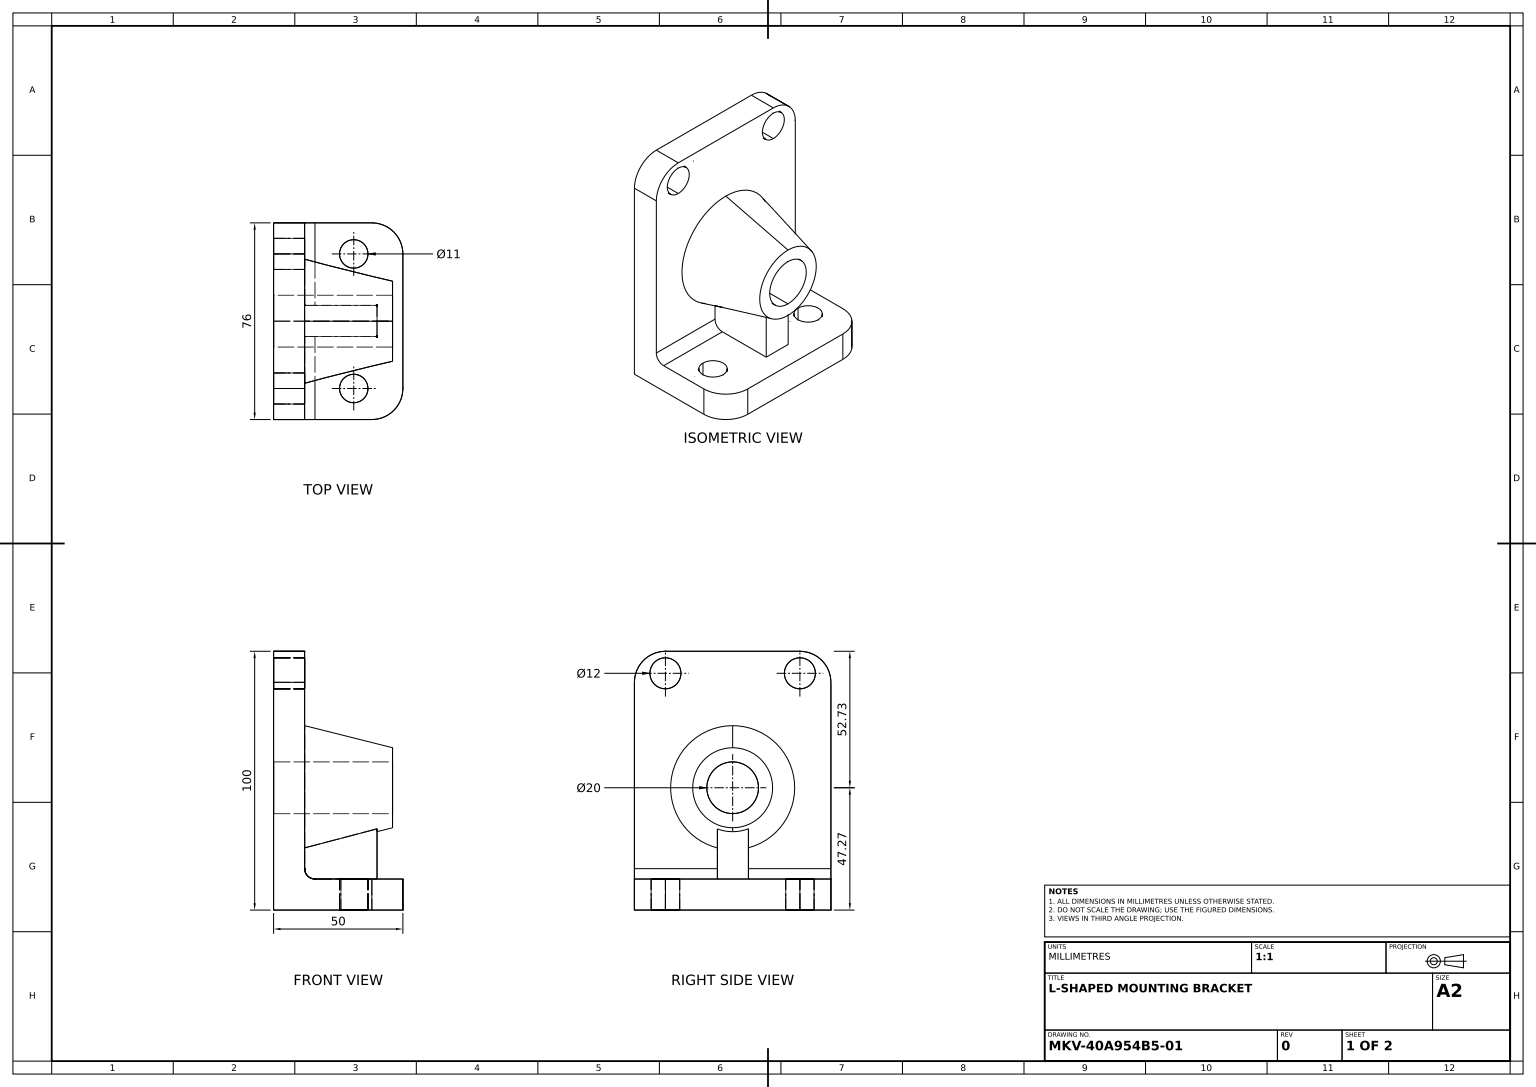
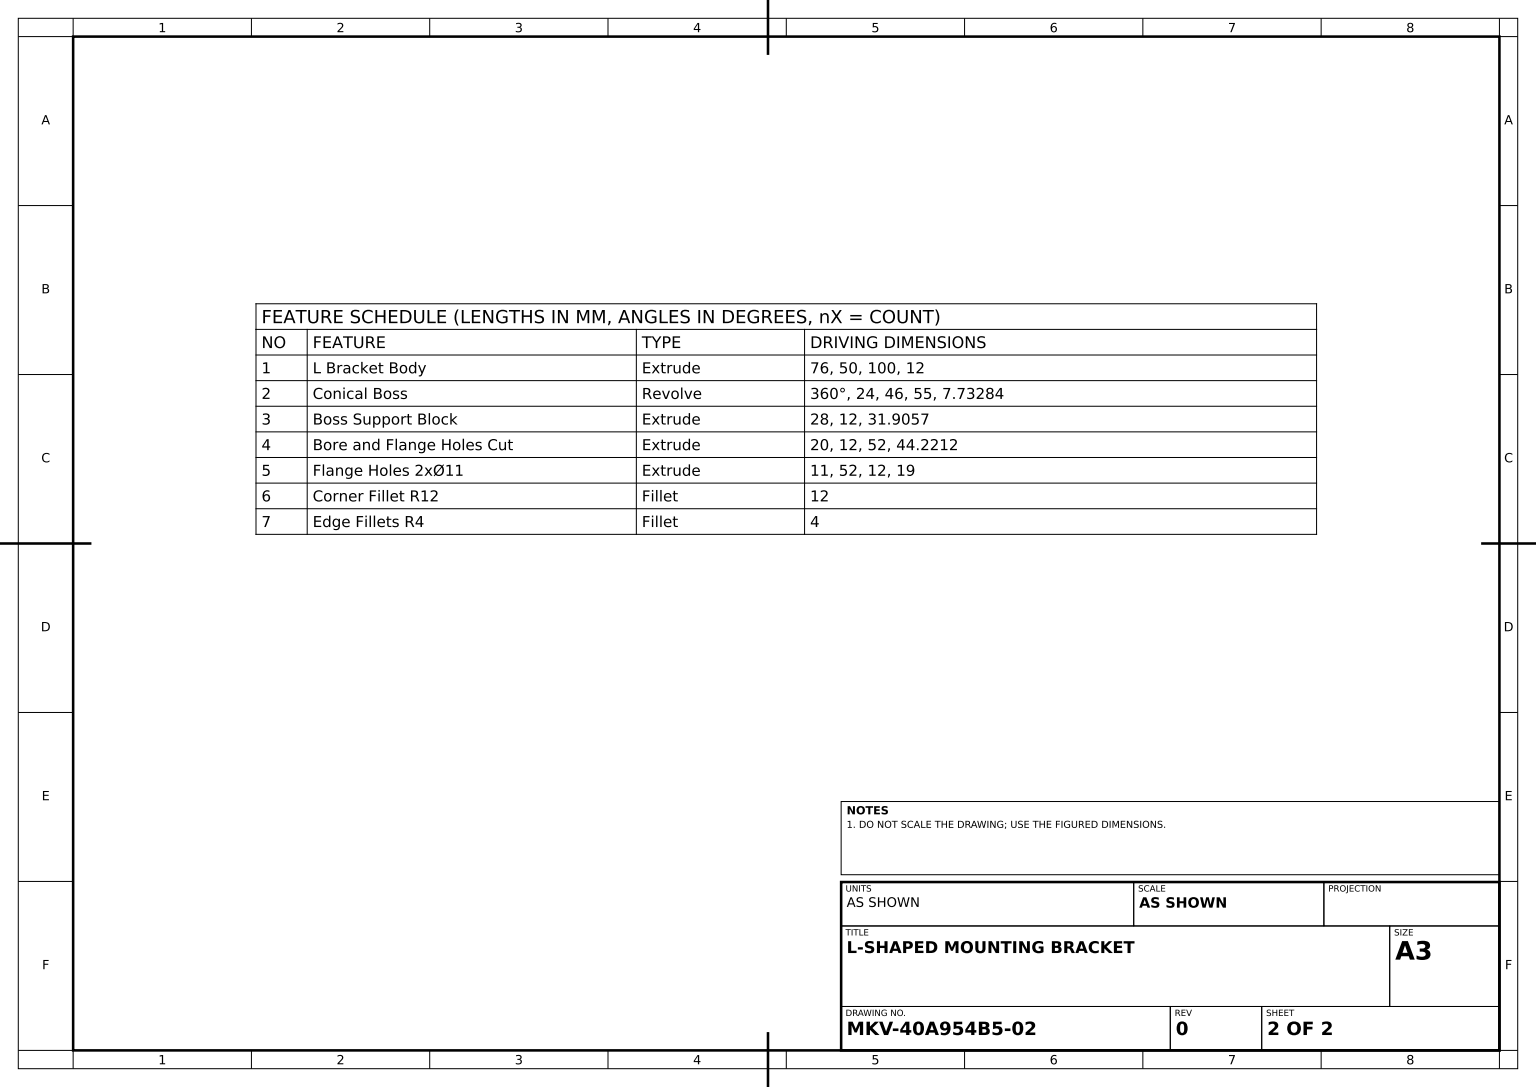
ISO-10303-21;
HEADER;
FILE_DESCRIPTION((''),'2;1');
FILE_NAME('','',(''),(''),'','','');
FILE_SCHEMA(('AUTOMOTIVE_DESIGN'));
ENDSEC;
DATA;
#1=APPLICATION_CONTEXT('');
#2=PRODUCT_CONTEXT('',#1,'mechanical');
#3=PRODUCT('','','',(#2));
#4=PRODUCT_DEFINITION_FORMATION('','',#3);
#5=PRODUCT_DEFINITION_CONTEXT('',#1,'design');
#6=PRODUCT_DEFINITION('','',#4,#5);
#7=PRODUCT_DEFINITION_SHAPE('','',#6);
#8=(LENGTH_UNIT()NAMED_UNIT(*)SI_UNIT(.MILLI.,.METRE.));
#9=(NAMED_UNIT(*)PLANE_ANGLE_UNIT()SI_UNIT($,.RADIAN.));
#10=(NAMED_UNIT(*)SI_UNIT($,.STERADIAN.)SOLID_ANGLE_UNIT());
#11=UNCERTAINTY_MEASURE_WITH_UNIT(LENGTH_MEASURE(1.E-05),#8,'distance_accuracy_value','');
#12=(GEOMETRIC_REPRESENTATION_CONTEXT(3)GLOBAL_UNCERTAINTY_ASSIGNED_CONTEXT((#11))GLOBAL_UNIT_ASSIGNED_CONTEXT((#8,#9,#10))REPRESENTATION_CONTEXT('',''));
#13=CARTESIAN_POINT('',(0.,57.267161,0.));
#14=VERTEX_POINT('',#13);
#15=CARTESIAN_POINT('',(46.,57.267161,0.));
#16=VERTEX_POINT('',#15);
#17=DIRECTION('',(1.,0.,0.));
#18=VECTOR('',#17,1000.);
#19=LINE('',#13,#18);
#20=EDGE_CURVE('',#14,#16,#19,.T.);
#21=ORIENTED_EDGE('',*,*,#20,.T.);
#22=CARTESIAN_POINT('',(46.,37.267161,0.));
#23=VERTEX_POINT('',#22);
#24=CARTESIAN_POINT('',(46.,47.267161,0.));
#25=DIRECTION('',(0.,1.,0.));
#26=AXIS2_PLACEMENT_3D('',#24,#17,#25);
#27=CIRCLE('',#26,10.);
#28=EDGE_CURVE('',#16,#23,#27,.T.);
#29=ORIENTED_EDGE('',*,*,#28,.T.);
#30=CARTESIAN_POINT('',(0.,37.267161,0.));
#31=VERTEX_POINT('',#30);
#32=LINE('',#30,#18);
#33=EDGE_CURVE('',#31,#23,#32,.T.);
#34=ORIENTED_EDGE('',*,*,#33,.F.);
#35=CARTESIAN_POINT('',(0.,47.267161,0.));
#36=AXIS2_PLACEMENT_3D('',#35,#17,#25);
#37=CIRCLE('',#36,10.);
#38=EDGE_CURVE('',#14,#31,#37,.T.);
#39=ORIENTED_EDGE('',*,*,#38,.F.);
#40=EDGE_LOOP('',(#21,#29,#34,#39));
#41=FACE_OUTER_BOUND('',#40,.T.);
#42=CYLINDRICAL_SURFACE('',#36,10.);
#43=ADVANCED_FACE('',(#41),#42,.F.);
#44=CARTESIAN_POINT('',(36.5,12.,-26.));
#45=VERTEX_POINT('',#44);
#46=CARTESIAN_POINT('',(25.5,12.,-26.));
#47=VERTEX_POINT('',#46);
#48=CARTESIAN_POINT('',(31.,12.,-26.));
#49=DIRECTION('',(-1.,0.,0.));
#50=AXIS2_PLACEMENT_3D('',#48,#25,#49);
#51=CIRCLE('',#50,5.5);
#52=EDGE_CURVE('',#45,#47,#51,.T.);
#53=ORIENTED_EDGE('',*,*,#52,.F.);
#54=EDGE_CURVE('',#47,#45,#51,.T.);
#55=ORIENTED_EDGE('',*,*,#54,.F.);
#56=EDGE_LOOP('',(#53,#55));
#57=FACE_BOUND('',#56,.T.);
#58=CARTESIAN_POINT('',(38.,12.,-38.));
#59=VERTEX_POINT('',#58);
#60=CARTESIAN_POINT('',(16.,12.,-38.));
#61=VERTEX_POINT('',#60);
#62=CARTESIAN_POINT('',(50.,12.,-38.));
#63=VECTOR('',#49,1000.);
#64=LINE('',#62,#63);
#65=EDGE_CURVE('',#59,#61,#64,.T.);
#66=ORIENTED_EDGE('',*,*,#65,.T.);
#67=CARTESIAN_POINT('',(16.,12.,-6.094262));
#68=VERTEX_POINT('',#67);
#69=DIRECTION('',(0.,0.,1.));
#70=VECTOR('',#69,1000.);
#71=LINE('',#67,#70);
#72=EDGE_CURVE('',#61,#68,#71,.T.);
#73=ORIENTED_EDGE('',*,*,#72,.T.);
#74=CARTESIAN_POINT('',(40.,12.,-6.094262));
#75=VERTEX_POINT('',#74);
#76=CARTESIAN_POINT('',(12.,12.,-6.094262));
#77=LINE('',#76,#18);
#78=EDGE_CURVE('',#68,#75,#77,.T.);
#79=ORIENTED_EDGE('',*,*,#78,.T.);
#80=CARTESIAN_POINT('',(40.,12.,5.905738));
#81=VERTEX_POINT('',#80);
#82=DIRECTION('',(0.,0.,-1.));
#83=VECTOR('',#82,1000.);
#84=LINE('',#80,#83);
#85=EDGE_CURVE('',#81,#75,#84,.T.);
#86=ORIENTED_EDGE('',*,*,#85,.F.);
#87=CARTESIAN_POINT('',(16.,12.,5.905738));
#88=VERTEX_POINT('',#87);
#89=CARTESIAN_POINT('',(12.,12.,5.905738));
#90=LINE('',#89,#18);
#91=EDGE_CURVE('',#88,#81,#90,.T.);
#92=ORIENTED_EDGE('',*,*,#91,.F.);
#93=CARTESIAN_POINT('',(16.,12.,38.));
#94=VERTEX_POINT('',#93);
#95=LINE('',#93,#70);
#96=EDGE_CURVE('',#88,#94,#95,.T.);
#97=ORIENTED_EDGE('',*,*,#96,.T.);
#98=CARTESIAN_POINT('',(38.,12.,38.));
#99=VERTEX_POINT('',#98);
#100=CARTESIAN_POINT('',(50.,12.,38.));
#101=LINE('',#100,#63);
#102=EDGE_CURVE('',#99,#94,#101,.T.);
#103=ORIENTED_EDGE('',*,*,#102,.F.);
#104=CARTESIAN_POINT('',(50.,12.,26.));
#105=VERTEX_POINT('',#104);
#106=CARTESIAN_POINT('',(38.,12.,26.));
#107=AXIS2_PLACEMENT_3D('',#106,#25,#17);
#108=CIRCLE('',#107,12.);
#109=EDGE_CURVE('',#99,#105,#108,.T.);
#110=ORIENTED_EDGE('',*,*,#109,.T.);
#111=CARTESIAN_POINT('',(50.,12.,-26.));
#112=VERTEX_POINT('',#111);
#113=LINE('',#100,#83);
#114=EDGE_CURVE('',#105,#112,#113,.T.);
#115=ORIENTED_EDGE('',*,*,#114,.T.);
#116=CARTESIAN_POINT('',(38.,12.,-26.));
#117=AXIS2_PLACEMENT_3D('',#116,#25,#17);
#118=CIRCLE('',#117,12.);
#119=EDGE_CURVE('',#112,#59,#118,.T.);
#120=ORIENTED_EDGE('',*,*,#119,.T.);
#121=EDGE_LOOP('',(#66,#73,#79,#86,#92,#97,#103,#110,#115,#120));
#122=FACE_OUTER_BOUND('',#121,.T.);
#123=CARTESIAN_POINT('',(36.5,12.,26.));
#124=VERTEX_POINT('',#123);
#125=CARTESIAN_POINT('',(25.5,12.,26.));
#126=VERTEX_POINT('',#125);
#127=CARTESIAN_POINT('',(31.,12.,26.));
#128=AXIS2_PLACEMENT_3D('',#127,#25,#49);
#129=CIRCLE('',#128,5.5);
#130=EDGE_CURVE('',#124,#126,#129,.T.);
#131=ORIENTED_EDGE('',*,*,#130,.F.);
#132=EDGE_CURVE('',#126,#124,#129,.T.);
#133=ORIENTED_EDGE('',*,*,#132,.F.);
#134=EDGE_LOOP('',(#131,#133));
#135=FACE_BOUND('',#134,.T.);
#136=DIRECTION('',(0.,-1.,0.));
#137=AXIS2_PLACEMENT_3D('',#100,#136,#17);
#138=PLANE('',#137);
#139=ADVANCED_FACE('',(#57,#122,#135),#138,.F.);
#140=CARTESIAN_POINT('',(50.,0.,-26.));
#141=VERTEX_POINT('',#140);
#142=VECTOR('',#25,1000.);
#143=LINE('',#140,#142);
#144=EDGE_CURVE('',#141,#112,#143,.T.);
#145=ORIENTED_EDGE('',*,*,#144,.T.);
#146=ORIENTED_EDGE('',*,*,#114,.F.);
#147=CARTESIAN_POINT('',(50.,0.,26.));
#148=VERTEX_POINT('',#147);
#149=VECTOR('',#136,1000.);
#150=LINE('',#147,#149);
#151=EDGE_CURVE('',#105,#148,#150,.T.);
#152=ORIENTED_EDGE('',*,*,#151,.T.);
#153=CARTESIAN_POINT('',(50.,0.,38.));
#154=LINE('',#153,#83);
#155=EDGE_CURVE('',#148,#141,#154,.T.);
#156=ORIENTED_EDGE('',*,*,#155,.T.);
#157=EDGE_LOOP('',(#145,#146,#152,#156));
#158=FACE_OUTER_BOUND('',#157,.T.);
#159=AXIS2_PLACEMENT_3D('',#153,#49,#69);
#160=PLANE('',#159);
#161=ADVANCED_FACE('',(#158),#160,.F.);
#162=CARTESIAN_POINT('',(0.,88.,-38.));
#163=VERTEX_POINT('',#162);
#164=CARTESIAN_POINT('',(12.,88.,-38.));
#165=VERTEX_POINT('',#164);
#166=LINE('',#162,#18);
#167=EDGE_CURVE('',#163,#165,#166,.T.);
#168=ORIENTED_EDGE('',*,*,#167,.F.);
#169=CARTESIAN_POINT('',(0.,100.,-26.));
#170=VERTEX_POINT('',#169);
#171=CARTESIAN_POINT('',(0.,88.,-26.));
#172=AXIS2_PLACEMENT_3D('',#171,#49,#25);
#173=CIRCLE('',#172,12.);
#174=EDGE_CURVE('',#170,#163,#173,.T.);
#175=ORIENTED_EDGE('',*,*,#174,.F.);
#176=CARTESIAN_POINT('',(12.,100.,-26.));
#177=VERTEX_POINT('',#176);
#178=LINE('',#176,#63);
#179=EDGE_CURVE('',#177,#170,#178,.T.);
#180=ORIENTED_EDGE('',*,*,#179,.F.);
#181=CARTESIAN_POINT('',(12.,88.,-26.));
#182=AXIS2_PLACEMENT_3D('',#181,#17,#136);
#183=CIRCLE('',#182,12.);
#184=EDGE_CURVE('',#165,#177,#183,.T.);
#185=ORIENTED_EDGE('',*,*,#184,.F.);
#186=EDGE_LOOP('',(#168,#175,#180,#185));
#187=FACE_OUTER_BOUND('',#186,.T.);
#188=AXIS2_PLACEMENT_3D('',#181,#49,#69);
#189=CYLINDRICAL_SURFACE('',#188,12.);
#190=ADVANCED_FACE('',(#187),#189,.T.);
#191=CARTESIAN_POINT('',(40.,31.356095,5.905738));
#192=VERTEX_POINT('',#191);
#193=CARTESIAN_POINT('',(40.,100.001,5.905738));
#194=LINE('',#193,#149);
#195=EDGE_CURVE('',#192,#81,#194,.T.);
#196=ORIENTED_EDGE('',*,*,#195,.T.);
#197=ORIENTED_EDGE('',*,*,#85,.T.);
#198=CARTESIAN_POINT('',(40.,31.427346,-6.094262));
#199=VERTEX_POINT('',#198);
#200=CARTESIAN_POINT('',(40.,100.001,-6.094262));
#201=LINE('',#200,#149);
#202=EDGE_CURVE('',#199,#75,#201,.T.);
#203=ORIENTED_EDGE('',*,*,#202,.F.);
#204=CARTESIAN_POINT('',(40.,30.295426,0.));
#205=VERTEX_POINT('',#204);
#206=CARTESIAN_POINT('',(40.,47.267161,0.));
#207=AXIS2_PLACEMENT_3D('',#206,#49,#136);
#208=CIRCLE('',#207,16.971735);
#209=EDGE_CURVE('',#199,#205,#208,.T.);
#210=ORIENTED_EDGE('',*,*,#209,.T.);
#211=EDGE_CURVE('',#205,#192,#208,.T.);
#212=ORIENTED_EDGE('',*,*,#211,.T.);
#213=EDGE_LOOP('',(#196,#197,#203,#210,#212));
#214=FACE_OUTER_BOUND('',#213,.T.);
#215=AXIS2_PLACEMENT_3D('',#193,#49,#136);
#216=PLANE('',#215);
#217=ADVANCED_FACE('',(#214),#216,.F.);
#218=CARTESIAN_POINT('',(0.,85.488396,26.));
#219=VERTEX_POINT('',#218);
#220=CARTESIAN_POINT('',(12.,85.488396,26.));
#221=VERTEX_POINT('',#220);
#222=LINE('',#218,#18);
#223=EDGE_CURVE('',#219,#221,#222,.T.);
#224=ORIENTED_EDGE('',*,*,#223,.T.);
#225=CARTESIAN_POINT('',(12.,97.488396,26.));
#226=VERTEX_POINT('',#225);
#227=CARTESIAN_POINT('',(12.,91.488396,26.));
#228=AXIS2_PLACEMENT_3D('',#227,#49,#136);
#229=CIRCLE('',#228,6.);
#230=EDGE_CURVE('',#226,#221,#229,.T.);
#231=ORIENTED_EDGE('',*,*,#230,.F.);
#232=CARTESIAN_POINT('',(0.,97.488396,26.));
#233=VERTEX_POINT('',#232);
#234=LINE('',#232,#18);
#235=EDGE_CURVE('',#233,#226,#234,.T.);
#236=ORIENTED_EDGE('',*,*,#235,.F.);
#237=CARTESIAN_POINT('',(0.,91.488396,26.));
#238=AXIS2_PLACEMENT_3D('',#237,#17,#25);
#239=CIRCLE('',#238,6.);
#240=EDGE_CURVE('',#219,#233,#239,.T.);
#241=ORIENTED_EDGE('',*,*,#240,.F.);
#242=EDGE_LOOP('',(#224,#231,#236,#241));
#243=FACE_OUTER_BOUND('',#242,.T.);
#244=CYLINDRICAL_SURFACE('',#238,6.);
#245=ADVANCED_FACE('',(#243),#244,.F.);
#246=EDGE_CURVE('',#221,#226,#229,.T.);
#247=ORIENTED_EDGE('',*,*,#246,.F.);
#248=ORIENTED_EDGE('',*,*,#223,.F.);
#249=EDGE_CURVE('',#233,#219,#239,.T.);
#250=ORIENTED_EDGE('',*,*,#249,.F.);
#251=ORIENTED_EDGE('',*,*,#235,.T.);
#252=EDGE_LOOP('',(#247,#248,#250,#251));
#253=FACE_OUTER_BOUND('',#252,.T.);
#254=ADVANCED_FACE('',(#253),#244,.F.);
#255=CARTESIAN_POINT('',(46.,31.801483,0.));
#256=VERTEX_POINT('',#255);
#257=CARTESIAN_POINT('',(46.,62.732839,0.));
#258=VERTEX_POINT('',#257);
#259=CIRCLE('',#26,15.465678);
#260=EDGE_CURVE('',#256,#258,#259,.T.);
#261=ORIENTED_EDGE('',*,*,#260,.T.);
#262=EDGE_CURVE('',#258,#256,#259,.T.);
#263=ORIENTED_EDGE('',*,*,#262,.T.);
#264=EDGE_LOOP('',(#261,#263));
#265=FACE_OUTER_BOUND('',#264,.T.);
#266=EDGE_CURVE('',#23,#16,#27,.T.);
#267=ORIENTED_EDGE('',*,*,#266,.F.);
#268=ORIENTED_EDGE('',*,*,#28,.F.);
#269=EDGE_LOOP('',(#267,#268));
#270=FACE_BOUND('',#269,.T.);
#271=AXIS2_PLACEMENT_3D('',#257,#17,#25);
#272=PLANE('',#271);
#273=ADVANCED_FACE('',(#265,#270),#272,.T.);
#274=CARTESIAN_POINT('',(0.,97.488396,-26.));
#275=VERTEX_POINT('',#274);
#276=CARTESIAN_POINT('',(12.,97.488396,-26.));
#277=VERTEX_POINT('',#276);
#278=LINE('',#274,#18);
#279=EDGE_CURVE('',#275,#277,#278,.T.);
#280=ORIENTED_EDGE('',*,*,#279,.F.);
#281=CARTESIAN_POINT('',(0.,85.488396,-26.));
#282=VERTEX_POINT('',#281);
#283=CARTESIAN_POINT('',(0.,91.488396,-26.));
#284=AXIS2_PLACEMENT_3D('',#283,#17,#25);
#285=CIRCLE('',#284,6.);
#286=EDGE_CURVE('',#282,#275,#285,.T.);
#287=ORIENTED_EDGE('',*,*,#286,.F.);
#288=CARTESIAN_POINT('',(12.,85.488396,-26.));
#289=VERTEX_POINT('',#288);
#290=LINE('',#281,#18);
#291=EDGE_CURVE('',#282,#289,#290,.T.);
#292=ORIENTED_EDGE('',*,*,#291,.T.);
#293=CARTESIAN_POINT('',(12.,91.488396,-26.));
#294=AXIS2_PLACEMENT_3D('',#293,#49,#136);
#295=CIRCLE('',#294,6.);
#296=EDGE_CURVE('',#277,#289,#295,.T.);
#297=ORIENTED_EDGE('',*,*,#296,.F.);
#298=EDGE_LOOP('',(#280,#287,#292,#297));
#299=FACE_OUTER_BOUND('',#298,.T.);
#300=CYLINDRICAL_SURFACE('',#284,6.);
#301=ADVANCED_FACE('',(#299),#300,.F.);
#302=CARTESIAN_POINT('',(0.,88.,38.));
#303=VERTEX_POINT('',#302);
#304=CARTESIAN_POINT('',(0.,0.,38.));
#305=VERTEX_POINT('',#304);
#306=CARTESIAN_POINT('',(0.,100.,38.));
#307=LINE('',#306,#149);
#308=EDGE_CURVE('',#303,#305,#307,.T.);
#309=ORIENTED_EDGE('',*,*,#308,.T.);
#310=CARTESIAN_POINT('',(38.,0.,38.));
#311=VERTEX_POINT('',#310);
#312=LINE('',#304,#18);
#313=EDGE_CURVE('',#305,#311,#312,.T.);
#314=ORIENTED_EDGE('',*,*,#313,.T.);
#315=LINE('',#98,#142);
#316=EDGE_CURVE('',#311,#99,#315,.T.);
#317=ORIENTED_EDGE('',*,*,#316,.T.);
#318=ORIENTED_EDGE('',*,*,#102,.T.);
#319=CARTESIAN_POINT('',(12.,16.,38.));
#320=VERTEX_POINT('',#319);
#321=CARTESIAN_POINT('',(16.,16.,38.));
#322=AXIS2_PLACEMENT_3D('',#321,#82,#17);
#323=CIRCLE('',#322,4.);
#324=EDGE_CURVE('',#94,#320,#323,.T.);
#325=ORIENTED_EDGE('',*,*,#324,.T.);
#326=CARTESIAN_POINT('',(12.,88.,38.));
#327=VERTEX_POINT('',#326);
#328=CARTESIAN_POINT('',(12.,12.,38.));
#329=LINE('',#328,#142);
#330=EDGE_CURVE('',#320,#327,#329,.T.);
#331=ORIENTED_EDGE('',*,*,#330,.T.);
#332=LINE('',#302,#63);
#333=EDGE_CURVE('',#327,#303,#332,.T.);
#334=ORIENTED_EDGE('',*,*,#333,.T.);
#335=EDGE_LOOP('',(#309,#314,#317,#318,#325,#331,#334));
#336=FACE_OUTER_BOUND('',#335,.T.);
#337=AXIS2_PLACEMENT_3D('',#304,#69,#17);
#338=PLANE('',#337);
#339=ADVANCED_FACE('',(#336),#338,.T.);
#340=CARTESIAN_POINT('',(12.,71.267161,0.));
#341=VERTEX_POINT('',#340);
#342=CARTESIAN_POINT('',(12.,24.005126,5.905738));
#343=VERTEX_POINT('',#342);
#344=CARTESIAN_POINT('',(12.,47.267161,0.));
#345=AXIS2_PLACEMENT_3D('',#344,#17,#25);
#346=CIRCLE('',#345,24.);
#347=EDGE_CURVE('',#341,#343,#346,.T.);
#348=ORIENTED_EDGE('',*,*,#347,.F.);
#349=CARTESIAN_POINT('',(12.,24.053803,-6.094262));
#350=VERTEX_POINT('',#349);
#351=EDGE_CURVE('',#350,#341,#346,.T.);
#352=ORIENTED_EDGE('',*,*,#351,.F.);
#353=CARTESIAN_POINT('',(12.,16.,-6.094262));
#354=VERTEX_POINT('',#353);
#355=CARTESIAN_POINT('',(12.,100.001,-6.094262));
#356=LINE('',#355,#149);
#357=EDGE_CURVE('',#350,#354,#356,.T.);
#358=ORIENTED_EDGE('',*,*,#357,.T.);
#359=CARTESIAN_POINT('',(12.,16.,-38.));
#360=VERTEX_POINT('',#359);
#361=LINE('',#359,#83);
#362=EDGE_CURVE('',#354,#360,#361,.T.);
#363=ORIENTED_EDGE('',*,*,#362,.T.);
#364=CARTESIAN_POINT('',(12.,12.,-38.));
#365=LINE('',#364,#142);
#366=EDGE_CURVE('',#360,#165,#365,.T.);
#367=ORIENTED_EDGE('',*,*,#366,.T.);
#368=ORIENTED_EDGE('',*,*,#184,.T.);
#369=CARTESIAN_POINT('',(12.,100.,26.));
#370=VERTEX_POINT('',#369);
#371=CARTESIAN_POINT('',(12.,100.,38.));
#372=LINE('',#371,#83);
#373=EDGE_CURVE('',#370,#177,#372,.T.);
#374=ORIENTED_EDGE('',*,*,#373,.F.);
#375=CARTESIAN_POINT('',(12.,88.,26.));
#376=AXIS2_PLACEMENT_3D('',#375,#17,#136);
#377=CIRCLE('',#376,12.);
#378=EDGE_CURVE('',#370,#327,#377,.T.);
#379=ORIENTED_EDGE('',*,*,#378,.T.);
#380=ORIENTED_EDGE('',*,*,#330,.F.);
#381=CARTESIAN_POINT('',(12.,16.,5.905738));
#382=VERTEX_POINT('',#381);
#383=LINE('',#381,#83);
#384=EDGE_CURVE('',#320,#382,#383,.T.);
#385=ORIENTED_EDGE('',*,*,#384,.T.);
#386=CARTESIAN_POINT('',(12.,100.001,5.905738));
#387=LINE('',#386,#149);
#388=EDGE_CURVE('',#343,#382,#387,.T.);
#389=ORIENTED_EDGE('',*,*,#388,.F.);
#390=EDGE_LOOP('',(#348,#352,#358,#363,#367,#368,#374,#379,#380,#385,#389));
#391=FACE_OUTER_BOUND('',#390,.T.);
#392=ORIENTED_EDGE('',*,*,#296,.T.);
#393=EDGE_CURVE('',#289,#277,#295,.T.);
#394=ORIENTED_EDGE('',*,*,#393,.T.);
#395=EDGE_LOOP('',(#392,#394));
#396=FACE_BOUND('',#395,.T.);
#397=ORIENTED_EDGE('',*,*,#230,.T.);
#398=ORIENTED_EDGE('',*,*,#246,.T.);
#399=EDGE_LOOP('',(#397,#398));
#400=FACE_BOUND('',#399,.T.);
#401=AXIS2_PLACEMENT_3D('',#328,#49,#136);
#402=PLANE('',#401);
#403=ADVANCED_FACE('',(#391,#396,#400),#402,.F.);
#404=ORIENTED_EDGE('',*,*,#179,.T.);
#405=CARTESIAN_POINT('',(0.,100.,26.));
#406=VERTEX_POINT('',#405);
#407=LINE('',#306,#83);
#408=EDGE_CURVE('',#406,#170,#407,.T.);
#409=ORIENTED_EDGE('',*,*,#408,.F.);
#410=LINE('',#369,#18);
#411=EDGE_CURVE('',#406,#370,#410,.T.);
#412=ORIENTED_EDGE('',*,*,#411,.T.);
#413=ORIENTED_EDGE('',*,*,#373,.T.);
#414=EDGE_LOOP('',(#404,#409,#412,#413));
#415=FACE_OUTER_BOUND('',#414,.T.);
#416=AXIS2_PLACEMENT_3D('',#371,#136,#82);
#417=PLANE('',#416);
#418=ADVANCED_FACE('',(#415),#417,.F.);
#419=ORIENTED_EDGE('',*,*,#316,.F.);
#420=CARTESIAN_POINT('',(38.,0.,26.));
#421=AXIS2_PLACEMENT_3D('',#420,#136,#69);
#422=CIRCLE('',#421,12.);
#423=EDGE_CURVE('',#148,#311,#422,.T.);
#424=ORIENTED_EDGE('',*,*,#423,.F.);
#425=ORIENTED_EDGE('',*,*,#151,.F.);
#426=ORIENTED_EDGE('',*,*,#109,.F.);
#427=EDGE_LOOP('',(#419,#424,#425,#426));
#428=FACE_OUTER_BOUND('',#427,.T.);
#429=AXIS2_PLACEMENT_3D('',#420,#136,#82);
#430=CYLINDRICAL_SURFACE('',#429,12.);
#431=ADVANCED_FACE('',(#428),#430,.T.);
#432=CARTESIAN_POINT('',(38.,0.,-38.));
#433=VERTEX_POINT('',#432);
#434=LINE('',#432,#149);
#435=EDGE_CURVE('',#59,#433,#434,.T.);
#436=ORIENTED_EDGE('',*,*,#435,.F.);
#437=ORIENTED_EDGE('',*,*,#119,.F.);
#438=ORIENTED_EDGE('',*,*,#144,.F.);
#439=CARTESIAN_POINT('',(38.,0.,-26.));
#440=AXIS2_PLACEMENT_3D('',#439,#136,#69);
#441=CIRCLE('',#440,12.);
#442=EDGE_CURVE('',#433,#141,#441,.T.);
#443=ORIENTED_EDGE('',*,*,#442,.F.);
#444=EDGE_LOOP('',(#436,#437,#438,#443));
#445=FACE_OUTER_BOUND('',#444,.T.);
#446=AXIS2_PLACEMENT_3D('',#439,#25,#69);
#447=CYLINDRICAL_SURFACE('',#446,12.);
#448=ADVANCED_FACE('',(#445),#447,.T.);
#449=ORIENTED_EDGE('',*,*,#209,.F.);
#450=CARTESIAN_POINT('',(35.339876,30.174021,-6.094262));
#451=CARTESIAN_POINT('',(30.675123,28.937928,-6.094262));
#452=CARTESIAN_POINT('',(21.340772,26.483787,-6.094262));
#453=CARTESIAN_POINT('',(16.671088,25.266023,-6.094262));
#454=B_SPLINE_CURVE_WITH_KNOTS('',3,(#198,#450,#451,#452,#453,#349),.UNSPECIFIED.,.F.,.F.,(4,2,4),(0.032304614,0.046780461,0.061256309),.UNSPECIFIED.);
#455=EDGE_CURVE('',#199,#350,#454,.T.);
#456=ORIENTED_EDGE('',*,*,#455,.T.);
#457=ORIENTED_EDGE('',*,*,#351,.T.);
#458=DIRECTION('',(-0.969911686,0.243457024,0.));
#459=VECTOR('',#458,1000.);
#460=LINE('',#257,#459);
#461=EDGE_CURVE('',#258,#341,#460,.T.);
#462=ORIENTED_EDGE('',*,*,#461,.F.);
#463=ORIENTED_EDGE('',*,*,#260,.F.);
#464=DIRECTION('',(-0.969911686,-0.243457024,0.));
#465=VECTOR('',#464,1000.);
#466=LINE('',#255,#465);
#467=EDGE_CURVE('',#256,#205,#466,.T.);
#468=ORIENTED_EDGE('',*,*,#467,.T.);
#469=EDGE_LOOP('',(#449,#456,#457,#462,#463,#468));
#470=FACE_OUTER_BOUND('',#469,.T.);
#471=AXIS2_PLACEMENT_3D('',#24,#49,#136);
#472=CONICAL_SURFACE('',#471,15.465677831,0.245928532);
#473=ADVANCED_FACE('',(#470),#472,.T.);
#474=CARTESIAN_POINT('',(16.,16.,-6.094262));
#475=AXIS2_PLACEMENT_3D('',#474,#82,#49);
#476=CIRCLE('',#475,4.);
#477=EDGE_CURVE('',#68,#354,#476,.T.);
#478=ORIENTED_EDGE('',*,*,#477,.F.);
#479=ORIENTED_EDGE('',*,*,#72,.F.);
#480=CARTESIAN_POINT('',(16.,16.,-38.));
#481=AXIS2_PLACEMENT_3D('',#480,#69,#17);
#482=CIRCLE('',#481,4.);
#483=EDGE_CURVE('',#360,#61,#482,.T.);
#484=ORIENTED_EDGE('',*,*,#483,.F.);
#485=ORIENTED_EDGE('',*,*,#362,.F.);
#486=EDGE_LOOP('',(#478,#479,#484,#485));
#487=FACE_OUTER_BOUND('',#486,.T.);
#488=AXIS2_PLACEMENT_3D('',#321,#69,#17);
#489=CYLINDRICAL_SURFACE('',#488,4.);
#490=ADVANCED_FACE('',(#487),#489,.F.);
#491=ORIENTED_EDGE('',*,*,#384,.F.);
#492=ORIENTED_EDGE('',*,*,#324,.F.);
#493=ORIENTED_EDGE('',*,*,#96,.F.);
#494=CARTESIAN_POINT('',(16.,16.,5.905738));
#495=AXIS2_PLACEMENT_3D('',#494,#69,#49);
#496=CIRCLE('',#495,4.);
#497=EDGE_CURVE('',#382,#88,#496,.T.);
#498=ORIENTED_EDGE('',*,*,#497,.F.);
#499=EDGE_LOOP('',(#491,#492,#493,#498));
#500=FACE_OUTER_BOUND('',#499,.T.);
#501=ADVANCED_FACE('',(#500),#489,.F.);
#502=CARTESIAN_POINT('',(35.339389,30.108252,5.905738));
#503=CARTESIAN_POINT('',(30.674502,28.876397,5.905738));
#504=CARTESIAN_POINT('',(21.340232,26.429505,5.905738));
#505=CARTESIAN_POINT('',(16.670771,25.214728,5.905738));
#506=B_SPLINE_CURVE_WITH_KNOTS('',3,(#191,#502,#503,#504,#505,#342),.UNSPECIFIED.,.F.,.F.,(4,2,4),(0.032313389,0.046786642,0.061259894),.UNSPECIFIED.);
#507=EDGE_CURVE('',#192,#343,#506,.T.);
#508=ORIENTED_EDGE('',*,*,#507,.T.);
#509=ORIENTED_EDGE('',*,*,#388,.T.);
#510=ORIENTED_EDGE('',*,*,#497,.T.);
#511=ORIENTED_EDGE('',*,*,#91,.T.);
#512=ORIENTED_EDGE('',*,*,#195,.F.);
#513=EDGE_LOOP('',(#508,#509,#510,#511,#512));
#514=FACE_OUTER_BOUND('',#513,.T.);
#515=AXIS2_PLACEMENT_3D('',#386,#82,#49);
#516=PLANE('',#515);
#517=ADVANCED_FACE('',(#514),#516,.F.);
#518=ORIENTED_EDGE('',*,*,#54,.T.);
#519=CARTESIAN_POINT('',(36.5,0.,-26.));
#520=VERTEX_POINT('',#519);
#521=LINE('',#519,#142);
#522=EDGE_CURVE('',#520,#45,#521,.T.);
#523=ORIENTED_EDGE('',*,*,#522,.F.);
#524=CARTESIAN_POINT('',(25.5,0.,-26.));
#525=VERTEX_POINT('',#524);
#526=CARTESIAN_POINT('',(31.,0.,-26.));
#527=AXIS2_PLACEMENT_3D('',#526,#25,#49);
#528=CIRCLE('',#527,5.5);
#529=EDGE_CURVE('',#525,#520,#528,.T.);
#530=ORIENTED_EDGE('',*,*,#529,.F.);
#531=LINE('',#524,#142);
#532=EDGE_CURVE('',#525,#47,#531,.T.);
#533=ORIENTED_EDGE('',*,*,#532,.T.);
#534=EDGE_LOOP('',(#518,#523,#530,#533));
#535=FACE_OUTER_BOUND('',#534,.T.);
#536=CYLINDRICAL_SURFACE('',#527,5.5);
#537=ADVANCED_FACE('',(#535),#536,.F.);
#538=ORIENTED_EDGE('',*,*,#529,.T.);
#539=EDGE_CURVE('',#520,#525,#528,.T.);
#540=ORIENTED_EDGE('',*,*,#539,.T.);
#541=EDGE_LOOP('',(#538,#540));
#542=FACE_BOUND('',#541,.T.);
#543=CARTESIAN_POINT('',(25.5,0.,26.));
#544=VERTEX_POINT('',#543);
#545=CARTESIAN_POINT('',(36.5,0.,26.));
#546=VERTEX_POINT('',#545);
#547=CARTESIAN_POINT('',(31.,0.,26.));
#548=AXIS2_PLACEMENT_3D('',#547,#25,#49);
#549=CIRCLE('',#548,5.5);
#550=EDGE_CURVE('',#544,#546,#549,.T.);
#551=ORIENTED_EDGE('',*,*,#550,.T.);
#552=EDGE_CURVE('',#546,#544,#549,.T.);
#553=ORIENTED_EDGE('',*,*,#552,.T.);
#554=EDGE_LOOP('',(#551,#553));
#555=FACE_BOUND('',#554,.T.);
#556=ORIENTED_EDGE('',*,*,#155,.F.);
#557=ORIENTED_EDGE('',*,*,#423,.T.);
#558=ORIENTED_EDGE('',*,*,#313,.F.);
#559=CARTESIAN_POINT('',(0.,0.,-38.));
#560=VERTEX_POINT('',#559);
#561=LINE('',#304,#83);
#562=EDGE_CURVE('',#305,#560,#561,.T.);
#563=ORIENTED_EDGE('',*,*,#562,.T.);
#564=LINE('',#559,#18);
#565=EDGE_CURVE('',#560,#433,#564,.T.);
#566=ORIENTED_EDGE('',*,*,#565,.T.);
#567=ORIENTED_EDGE('',*,*,#442,.T.);
#568=EDGE_LOOP('',(#556,#557,#558,#563,#566,#567));
#569=FACE_OUTER_BOUND('',#568,.T.);
#570=AXIS2_PLACEMENT_3D('',#304,#25,#69);
#571=PLANE('',#570);
#572=ADVANCED_FACE('',(#542,#555,#569),#571,.F.);
#573=ORIENTED_EDGE('',*,*,#33,.T.);
#574=ORIENTED_EDGE('',*,*,#266,.T.);
#575=ORIENTED_EDGE('',*,*,#20,.F.);
#576=EDGE_CURVE('',#31,#14,#37,.T.);
#577=ORIENTED_EDGE('',*,*,#576,.F.);
#578=EDGE_LOOP('',(#573,#574,#575,#577));
#579=FACE_OUTER_BOUND('',#578,.T.);
#580=ADVANCED_FACE('',(#579),#42,.F.);
#581=ORIENTED_EDGE('',*,*,#291,.F.);
#582=EDGE_CURVE('',#275,#282,#285,.T.);
#583=ORIENTED_EDGE('',*,*,#582,.F.);
#584=ORIENTED_EDGE('',*,*,#279,.T.);
#585=ORIENTED_EDGE('',*,*,#393,.F.);
#586=EDGE_LOOP('',(#581,#583,#584,#585));
#587=FACE_OUTER_BOUND('',#586,.T.);
#588=ADVANCED_FACE('',(#587),#300,.F.);
#589=LINE('',#545,#142);
#590=EDGE_CURVE('',#546,#124,#589,.T.);
#591=ORIENTED_EDGE('',*,*,#590,.T.);
#592=ORIENTED_EDGE('',*,*,#130,.T.);
#593=LINE('',#543,#142);
#594=EDGE_CURVE('',#544,#126,#593,.T.);
#595=ORIENTED_EDGE('',*,*,#594,.F.);
#596=ORIENTED_EDGE('',*,*,#552,.F.);
#597=EDGE_LOOP('',(#591,#592,#595,#596));
#598=FACE_OUTER_BOUND('',#597,.T.);
#599=CYLINDRICAL_SURFACE('',#548,5.5);
#600=ADVANCED_FACE('',(#598),#599,.F.);
#601=ORIENTED_EDGE('',*,*,#507,.F.);
#602=ORIENTED_EDGE('',*,*,#211,.F.);
#603=ORIENTED_EDGE('',*,*,#467,.F.);
#604=ORIENTED_EDGE('',*,*,#262,.F.);
#605=ORIENTED_EDGE('',*,*,#461,.T.);
#606=ORIENTED_EDGE('',*,*,#347,.T.);
#607=EDGE_LOOP('',(#601,#602,#603,#604,#605,#606));
#608=FACE_OUTER_BOUND('',#607,.T.);
#609=ADVANCED_FACE('',(#608),#472,.T.);
#610=ORIENTED_EDGE('',*,*,#78,.F.);
#611=ORIENTED_EDGE('',*,*,#477,.T.);
#612=ORIENTED_EDGE('',*,*,#357,.F.);
#613=ORIENTED_EDGE('',*,*,#455,.F.);
#614=ORIENTED_EDGE('',*,*,#202,.T.);
#615=EDGE_LOOP('',(#610,#611,#612,#613,#614));
#616=FACE_OUTER_BOUND('',#615,.T.);
#617=AXIS2_PLACEMENT_3D('',#355,#82,#49);
#618=PLANE('',#617);
#619=ADVANCED_FACE('',(#616),#618,.T.);
#620=ORIENTED_EDGE('',*,*,#378,.F.);
#621=ORIENTED_EDGE('',*,*,#411,.F.);
#622=CARTESIAN_POINT('',(0.,88.,26.));
#623=AXIS2_PLACEMENT_3D('',#622,#49,#25);
#624=CIRCLE('',#623,12.);
#625=EDGE_CURVE('',#303,#406,#624,.T.);
#626=ORIENTED_EDGE('',*,*,#625,.F.);
#627=ORIENTED_EDGE('',*,*,#333,.F.);
#628=EDGE_LOOP('',(#620,#621,#626,#627));
#629=FACE_OUTER_BOUND('',#628,.T.);
#630=AXIS2_PLACEMENT_3D('',#622,#17,#82);
#631=CYLINDRICAL_SURFACE('',#630,12.);
#632=ADVANCED_FACE('',(#629),#631,.T.);
#633=ORIENTED_EDGE('',*,*,#249,.T.);
#634=ORIENTED_EDGE('',*,*,#240,.T.);
#635=EDGE_LOOP('',(#633,#634));
#636=FACE_BOUND('',#635,.T.);
#637=ORIENTED_EDGE('',*,*,#38,.T.);
#638=ORIENTED_EDGE('',*,*,#576,.T.);
#639=EDGE_LOOP('',(#637,#638));
#640=FACE_BOUND('',#639,.T.);
#641=CARTESIAN_POINT('',(0.,100.,-38.));
#642=LINE('',#641,#149);
#643=EDGE_CURVE('',#163,#560,#642,.T.);
#644=ORIENTED_EDGE('',*,*,#643,.T.);
#645=ORIENTED_EDGE('',*,*,#562,.F.);
#646=ORIENTED_EDGE('',*,*,#308,.F.);
#647=ORIENTED_EDGE('',*,*,#625,.T.);
#648=ORIENTED_EDGE('',*,*,#408,.T.);
#649=ORIENTED_EDGE('',*,*,#174,.T.);
#650=EDGE_LOOP('',(#644,#645,#646,#647,#648,#649));
#651=FACE_OUTER_BOUND('',#650,.T.);
#652=ORIENTED_EDGE('',*,*,#582,.T.);
#653=ORIENTED_EDGE('',*,*,#286,.T.);
#654=EDGE_LOOP('',(#652,#653));
#655=FACE_BOUND('',#654,.T.);
#656=AXIS2_PLACEMENT_3D('',#306,#17,#25);
#657=PLANE('',#656);
#658=ADVANCED_FACE('',(#636,#640,#651,#655),#657,.F.);
#659=ORIENTED_EDGE('',*,*,#594,.T.);
#660=ORIENTED_EDGE('',*,*,#132,.T.);
#661=ORIENTED_EDGE('',*,*,#590,.F.);
#662=ORIENTED_EDGE('',*,*,#550,.F.);
#663=EDGE_LOOP('',(#659,#660,#661,#662));
#664=FACE_OUTER_BOUND('',#663,.T.);
#665=ADVANCED_FACE('',(#664),#599,.F.);
#666=ORIENTED_EDGE('',*,*,#532,.F.);
#667=ORIENTED_EDGE('',*,*,#539,.F.);
#668=ORIENTED_EDGE('',*,*,#522,.T.);
#669=ORIENTED_EDGE('',*,*,#52,.T.);
#670=EDGE_LOOP('',(#666,#667,#668,#669));
#671=FACE_OUTER_BOUND('',#670,.T.);
#672=ADVANCED_FACE('',(#671),#536,.F.);
#673=ORIENTED_EDGE('',*,*,#167,.T.);
#674=ORIENTED_EDGE('',*,*,#366,.F.);
#675=ORIENTED_EDGE('',*,*,#483,.T.);
#676=ORIENTED_EDGE('',*,*,#65,.F.);
#677=ORIENTED_EDGE('',*,*,#435,.T.);
#678=ORIENTED_EDGE('',*,*,#565,.F.);
#679=ORIENTED_EDGE('',*,*,#643,.F.);
#680=EDGE_LOOP('',(#673,#674,#675,#676,#677,#678,#679));
#681=FACE_OUTER_BOUND('',#680,.T.);
#682=AXIS2_PLACEMENT_3D('',#559,#69,#17);
#683=PLANE('',#682);
#684=ADVANCED_FACE('',(#681),#683,.F.);
#685=CLOSED_SHELL('',(#43,#139,#161,#190,#217,#245,#254,#273,#301,#339,#403,#418,#431,#448,#473,#490,#501,#517,#537,#572,#580,#588,#600,#609,#619,#632,#658,#665,#672,#684));
#686=MANIFOLD_SOLID_BREP('',#685);
#687=ADVANCED_BREP_SHAPE_REPRESENTATION('',(#686),#12);
#688=SHAPE_DEFINITION_REPRESENTATION(#7,#687);
ENDSEC;
END-ISO-10303-21;
